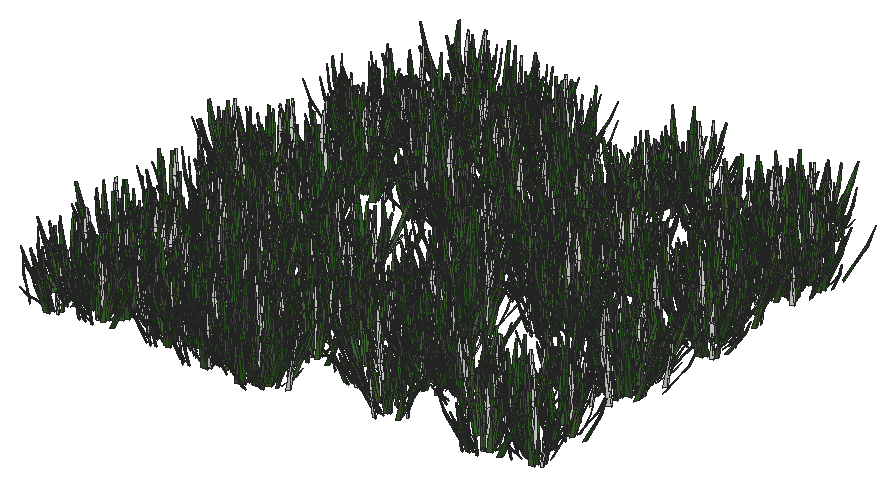
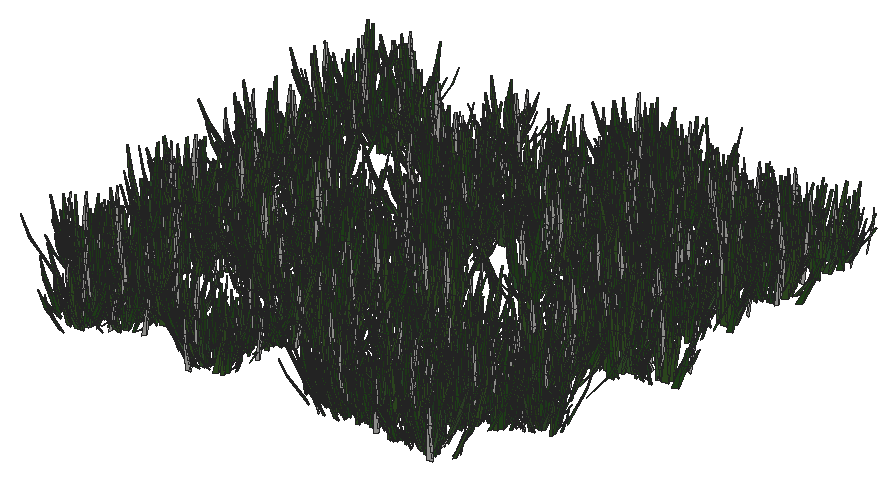
# SketchUp Ruby script. Lengths in inches.
U = 1.inch
M = Sketchup.active_model
def pt(a) = Geom::Point3d.new(a.map { |v| v * U })
def face(e, loops, mat)
  f = e.add_face(loops[0].map { |a| pt(a) })
  loops[1..].each { |l| e.add_face(l.map { |a| pt(a) }).erase! }
  f.material = f.back_material = mat if mat
  f
end
# faces: each face lists its corners as indices into pts; further lists are holes
def faces(e, pts, list, mat = nil) = list.each { |f| face(e, (f[0].is_a?(Array) ? f : [f]).map { |l| l.map { |i| pts[i] } }, mat) }
# xy, xz, yz: faces in a plane at the given z, y or x. An outline is a flat list of corners, or four numbers for a rectangle; further outlines are holes
def ring(l) = l.size == 4 ? [[l[0], l[1]], [l[2], l[1]], [l[2], l[3]], [l[0], l[3]]] : l.each_slice(2).to_a
def flat(e, list, mat, &to3) = list.each { |f| face(e, (f[0].is_a?(Array) ? f : [f]).map { |l| ring(l).map { |u, v| to3.(u, v) } }, mat) }
def xy(e, z, list, mat = nil) = flat(e, list, mat) { |x, y| [x, y, z] }
def xz(e, y, list, mat = nil) = flat(e, list, mat) { |x, z| [x, y, z] }
def yz(e, x, list, mat = nil) = flat(e, list, mat) { |y, z| [x, y, z] }
def lines(e, pts, list) = list.each { |a, b| e.add_line(pt(pts[a]), pt(pts[b])) }
# prism: a flat outline (further loops are holes) pulled along v
def prism(e, loops, v, mat = nil)
  f = face(e, loops, mat); d = Geom::Vector3d.new(v.map { |x| x * U })
  f.pushpull(f.normal.samedirection?(d) ? d.length : -d.length)
end
def box(e, o, s, mat = nil) = prism(e, [[o, [o[0] + s[0], o[1], o[2]], [o[0] + s[0], o[1] + s[1], o[2]], [o[0], o[1] + s[1], o[2]]]], [0, 0, s[2]], mat)
def at(x, y, z, deg = 0) = Geom::Transformation.translation(pt([x, y, z])) * Geom::Transformation.rotation(ORIGIN, Z_AXIS, deg.degrees)
def axes(o, x, y, z) = Geom::Transformation.new([*x, 0, *y, 0, *z, 0, *pt(o).to_a, 1])
def part(name) = M.definitions.add(name)
# library, detail: a bought-in or finely detailed component or shape, given as its bounding box
def library(name, o, s) = part(name).tap { |d| box(d.entities, o, s) }
def detail(e, o, s) = box(e.add_group.entities, o, s)
def put(e, d, t, mat = nil) = e.add_instance(d, t).tap { |i| i.material = mat if mat }
def group(e, t, mat = nil) = e.add_group.tap { |g| g.transformation = t; g.material = mat if mat }.entities
root = M.entities
M.materials.add("Material1").color = [58, 110, 58]
M.materials.add("Material10").color = [48, 100, 38]
M.materials.add("Material3").color = [68, 110, 58]
M.materials.add("Material4").color = [48, 90, 38]
M.materials.add("Material5").color = [68, 110, 48]
M.materials.add("Material6").color = [48, 90, 48]
M.materials.add("Material8").color = [58, 90, 38]
M.materials.add("Material9").color = [68, 100, 58]
c1 = part("grass00")
p = [[-0.6875,0.15,0],[-0.56,0.08,5.52],[-0.04,0.03,2.76],[0.48,-0.02,0],[0.35,-0.02,5.52],[-0.1,-0.14,5.52],
  [-0.12,0.65,8.37],[-0.42,0.65,8.37]]
faces(c1.entities,p,[[0,1,2,3],[3,2,4],[1,5,2],[5,4,2],[1,6,5],[4,5,6],[7,6,1]])
c2 = part("Group16\#1")
put(c2.entities,c1,axes([1.44,-0.61,-0.01],[0.05352,0.12609,0],[-0.10704,0.04543,0.07239],[0.06664,-0.02828,0.11628]),"Material6")
put(c2.entities,c1,axes([0.76,-0.15,-0.01],[0.04676,0.24062,0],[-0.23162,0.04501,0.06642],[0.0652,-0.01267,0.23595]),"Material3")
put(c2.entities,c1,axes([0.79,0.01,-0.01],[-0.00606,0.34651,0],[-0.34381,-0.00602,0.0432],[0.04319,0.00076,0.34386]))
put(c2.entities,c1,axes([1,0.23,-0.01],[-0.07192,0.31144,0],[-0.28722,-0.06632,0.1236],[0.12043,0.02781,0.29478]),"Material5")
put(c2.entities,c1,axes([1.66,0.77,-0.01],[-0.13828,0.29651,0],[-0.21551,-0.1005,0.22471],[0.20365,0.09498,0.23779]),"Material10")
put(c2.entities,c1,axes([0.6875,0.52,-0.01],[-0.18126,0.24051,0],[-0.22746,-0.17142,0.09788],[0.07817,0.05891,0.28481]),"Material5")
put(c2.entities,c1,axes([0.68,0.78,-0.01],[-0.215,0.18688,0],[-0.12385,-0.14248,0.21334],[0.13995,0.16101,0.18878]),"Material3")
put(c2.entities,c1,axes([0.56,1,-0.01],[-0.13756,0.07624,0],[-0.06159,-0.11112,0.0927],[0.04494,0.08108,0.12705]),"Material5")
put(c2.entities,c1,axes([0.2,0.64,-0.01],[-0.23729,0.07254,0],[-0.05711,-0.18681,0.153],[0.04473,0.14632,0.19535]),"Material10")
put(c2.entities,c1,axes([0.0625,0.72,-0.01],[-0.28874,0.02525,0],[-0.02179,-0.24916,0.14647],[0.01276,0.14591,0.25012]),"Material3")
put(c2.entities,c1,axes([-0.08,0.62,-0.01],[-0.34089,-0.04187,0],[0.03255,-0.26504,0.216],[-0.02633,0.21439,0.26703]),"Material10")
put(c2.entities,c1,axes([-0.34,0.98,-0.01],[-0.14314,-0.0493,0],[0.04397,-0.12769,0.06843],[-0.02228,0.0647,0.13505]),"Material10")
put(c2.entities,c1,axes([-0.87,1.45,-0.01],[-0.23488,-0.14114,0],[0.13761,-0.22901,0.06087],[-0.03135,0.05217,0.26717]))
put(c2.entities,c1,axes([-0.72,0.77,-0.01],[-0.14208,-0.13251,0],[0.07209,-0.0773,0.16301],[-0.11118,0.11922,0.1057]),"Material10")
put(c2.entities,c1,axes([-0.62,0.43,-0.01],[-0.14845,-0.21203,0],[0.18654,-0.13061,0.12304],[-0.10079,0.07057,0.22772]),"Material3")
put(c2.entities,c1,axes([-0.68,0.29,-0.01],[-0.13639,-0.32136,0],[0.31723,-0.13464,0.05579],[-0.05136,0.0218,0.34462]),"Material4")
put(c2.entities,c1,axes([-0.64,0.125,-0.01],[-0.0458,-0.23569,0],[0.22124,-0.043,0.08276],[-0.08124,0.01579,0.22538]),"Material1")
put(c2.entities,c1,axes([-1.6,-0.03,-0.01],[0.00576,-0.32897,0],[0.27526,0.00482,0.18018],[-0.18015,-0.00315,0.2753]),"Material5")
put(c2.entities,c1,axes([-1.36,-0.31,-0.01],[0.05718,-0.24765,0],[0.18172,0.04196,0.17267],[-0.16825,-0.03885,0.1865]),"Material10")
put(c2.entities,c1,axes([-1.54,-0.72,-0.01],[0.06537,-0.14017,0],[0.13555,0.06321,0.03939],[-0.0357,-0.01665,0.14956]))
put(c2.entities,c1,axes([-1.19,-0.9,-0.01],[0.09597,-0.12735,0],[0.11214,0.08451,0.07557],[-0.06035,-0.04548,0.14042]),"Material9")
put(c2.entities,c1,axes([-0.47,-0.54,-0.01],[0.11588,-0.10072,0],[0.0618,0.0711,0.12124],[-0.07953,-0.0915,0.0942]))
put(c2.entities,c1,axes([-0.47,-0.84,-0.01],[0.11927,-0.0661,0],[0.06603,0.11913,0.00646],[-0.00313,-0.00565,0.13621]),"Material5")
put(c2.entities,c1,axes([-0.38,-1.24,-0.01],[0.28037,-0.08571,0],[0.0618,0.20215,0.20315],[-0.05939,-0.19428,0.21139]),"Material9")
put(c2.entities,c1,axes([-0.06,-0.66,-0.01],[0.22719,-0.01987,0],[0.01247,0.14255,0.17758],[-0.01547,-0.17691,0.1431]),"Material8")
put(c2.entities,c1,axes([0.11,-0.89,-0.01],[0.14882,0.01828,0],[-0.01058,0.08611,0.12229],[0.01491,-0.12138,0.08676]),"Material6")
put(c2.entities,c1,axes([0.25,-0.72,-0.01],[0.20481,0.07053,0],[-0.06206,0.18022,0.10291],[0.03351,-0.0973,0.1906]),"Material6")
put(c2.entities,c1,axes([0.85,-1.42,-0.01],[0.16481,0.09904,0],[-0.09472,0.15762,0.05616],[0.02893,-0.04814,0.18389]),"Material5")
put(c2.entities,c1,axes([1.01,-1.09,-0.01],[0.21858,0.20385,0],[-0.17495,0.1876,0.15339],[0.10462,-0.11218,0.25652]),"Material10")
put(c2.entities,c1,axes([1.01,-0.71,-0.01],[0.08733,0.12473,0],[-0.06445,0.04512,0.13037],[0.1068,-0.07477,0.07867]),"Material6")
c3 = part("Group15\#1")
put(c3.entities,c2,at(0,0,0))
c4 = part("3darcstudiotree_grass00\#1")
put(c4.entities,c3,at(0,0,0))
put(root,c4,axes([313.43,128.25,0.25],[1.09323,-0.33647,0],[0.38565,0.86321,-0.01564],[0.00925,0.0207,1.88746]))
put(root,c4,axes([302.23,128.25,0.25],[0.61135,-0.6937,0],[0.76743,0.46592,-0.02877],[0.03641,0.02211,1.49076]))
put(root,c4,axes([310.46,128.14,0.25],[0.83193,0.6505,0],[-0.85398,0.75239,-0.01047],[-0.01109,0.00977,1.92288]))
put(root,c4,axes([314.96,128.14,0.25],[-0.65984,-0.73253,0],[0.79893,-0.49577,-0.02089],[0.02661,-0.01651,1.58683]))
put(root,c4,axes([299.16,128.03,0.25],[-0.33379,1.0049,0],[-0.95038,-0.21747,-0.03305],[-0.04366,-0.00999,1.35106]))
put(root,c4,axes([307.23,128.39,0.25],[0.52907,0.62243,0],[-0.7421,0.43455,-0.03223],[-0.03993,0.02338,1.37708]))
put(root,c4,axes([301.17,128.74,0.25],[1.04664,0.25601,0],[-0.25703,0.72391,-0.026],[-0.0129,0.03632,1.59572]))
put(root,c4,axes([311.2,128.65,0.25],[-1.02803,0.5315,0],[-0.48139,-0.64144,-0.01072],[-0.0115,-0.01532,1.84718]))
put(root,c4,axes([302.79,129.78,0.25],[1.1255,0.00235,0],[-0.00289,0.95262,-0.01268],[-0.00005,0.01678,1.83013]))
put(root,c4,axes([329.86,130.03,0.25],[0.62937,-0.55545,0],[0.77494,0.60491,-0.02136],[0.02372,0.01851,1.62144]))
put(root,c4,axes([310.44,129.93,0.25],[0.78925,0.37102,0],[-0.48273,0.70741,-0.02459],[-0.02361,0.0346,1.90817]))
put(root,c4,axes([299.36,129.74,0.25],[-0.10935,0.97509,0],[-1.19512,-0.09233,-0.02425],[-0.03553,-0.00274,1.76617]))
put(root,c4,axes([301.375,129.97,0.25],[0.27214,0.80157,0],[-1.04551,0.24453,-0.02067],[-0.03104,0.00726,1.69495]))
put(root,c4,axes([307.62,129.96,0.25],[0.12593,0.77017,0],[-0.97904,0.11028,-0.02967],[-0.04682,0.00527,1.57371]))
put(root,c4,axes([322.625,130.01,0.25],[-0.84483,0.43279,0],[-0.48176,-0.64786,-0.03387],[-0.02627,-0.03533,1.3548]))
put(root,c4,axes([305.28,130.84,0.25],[-0.84379,0.61822,0],[-0.85319,-0.80223,-0.01862],[-0.01823,-0.01715,1.90809]))
put(root,c4,axes([332.8125,131.04,0.25],[-0.49439,0.70839,0],[-0.82415,-0.39624,-0.02138],[-0.03174,-0.01526,1.63406]))
put(root,c4,axes([313.39,131.35,0.25],[-0.70228,-0.48257,0],[0.74708,-0.74899,-0.02106],[0.01665,-0.01669,1.45262]))
put(root,c4,axes([306.87,131.27,0.25],[-0.85735,0.46398,0],[-0.6008,-0.76479,-0.02083],[-0.01661,-0.02115,1.60618]))
put(root,c4,axes([301.49,131.9,0.25],[-0.71478,-0.65935,0],[0.79567,-0.59421,-0.02928],[0.02765,-0.02065,1.35967]))
put(root,c4,axes([311.6,132.11,0.25],[0.18112,-1.06483,0],[1.06399,0.12468,-0.01886],[0.0303,0.00355,1.74385]))
put(root,c4,axes([310.375,132.125,0.25],[1.08899,0.1057,0],[-0.112,0.79493,-0.0104],[-0.00234,0.01663,1.87036]))
put(root,c4,axes([304.09,132.35,0.25],[1.13568,-0.03992,0],[0.04696,0.92039,-0.02002],[0.00129,0.02535,1.69539]))
put(root,c4,axes([314.64,132.64,0.25],[0.8623,-0.69628,0],[0.62912,0.53673,-0.01443],[0.02081,0.01775,1.86565]))
put(root,c4,axes([318.99,132.49,0.25],[0.11272,1.05535,0],[-1.08573,0.07989,-0.0152],[-0.02232,0.00164,1.60635]))
put(root,c4,axes([322.37,133.39,0.25],[0.89828,0.57164,0],[-0.56596,0.61268,-0.03117],[-0.02658,0.02877,1.30357]))
put(root,c4,axes([325.61,133.9,0.25],[0.03302,-0.91614,0],[1.14545,0.02844,-0.01737],[0.02345,0.00058,1.54781]))
put(root,c4,axes([301.54,133.72,0.25],[-0.15265,0.9589,0],[-1.24925,-0.137,-0.03274],[-0.03717,-0.00408,1.44297]))
put(root,c4,axes([329.42,134.3,0.25],[0.89818,-0.35172,0],[0.49737,0.87499,-0.02435],[0.01511,0.02658,1.69455]))
put(root,c4,axes([311.57,133.92,0.25],[-1.14214,-0.02536,0],[0.03102,-0.96222,-0.01377],[0.00052,-0.01628,1.65227]))
put(root,c4,axes([299.1875,133.91,0.25],[-0.79807,0.55513,0],[-0.82006,-0.81217,-0.01682],[-0.01524,-0.01509,1.80026]))
put(root,c4,axes([332.37,134.4375,0.25],[0.86483,-0.466,0],[0.52618,0.67271,-0.02789],[0.02695,0.03446,1.71527]))
put(root,c4,axes([328.21,134.33,0.25],[-0.98544,0.42877,0],[-0.41843,-0.66251,-0.02232],[-0.01829,-0.02895,1.59039]))
put(root,c4,axes([302.13,134.41,0.25],[0.21228,0.86046,0],[-1.13808,0.19343,-0.02758],[-0.03776,0.00642,1.62317]))
put(root,c4,axes([299.88,134.7,0.25],[0.63523,0.53865,0],[-0.7856,0.63824,-0.01876],[-0.02159,0.01754,1.77063]))
put(root,c4,axes([309.61,135.07,0.25],[-0.08387,-0.77908,0],[1.1557,-0.08571,-0.01785],[0.02919,-0.00216,1.90542]))
put(root,c4,axes([320.69,134.98,0.25],[0.93635,0.57595,0],[-0.61403,0.6877,-0.03152],[-0.02685,0.03007,1.47514]))
put(root,c4,axes([321.74,135.15,0.25],[0.073,0.99528,0],[-1.03512,0.05231,-0.02381],[-0.04076,0.00206,1.77807]))
put(root,c4,axes([306.58,135.61,0.25],[-0.50394,-0.92094,0],[1.07294,-0.40446,-0.02239],[0.03283,-0.01238,1.89813]))
put(root,c4,axes([311.75,135.85,0.25],[1.04801,-0.5177,0],[0.58045,0.80949,-0.02674],[0.01812,0.02528,1.50406]))
put(root,c4,axes([305.66,136.03,0.25],[1.1531,0.08555,0],[-0.0892,0.82822,-0.01038],[-0.00179,0.01662,1.94021]))
put(root,c4,axes([308.67,135.98,0.25],[-0.82708,-0.3732,0],[0.44077,-0.67293,-0.02167],[0.01498,-0.02287,1.33527]))
put(root,c4,axes([322.77,135.96,0.25],[-1.19556,-0.39954,0],[0.44888,-0.92534,-0.01703],[0.00869,-0.01792,1.64249]))
put(root,c4,axes([314.28,136.01,0.25],[-1.04881,0.00914,0],[-0.01096,-0.86641,-0.01485],[-0.00024,-0.01921,1.62647]))
put(root,c4,axes([315.67,136.35,0.25],[-0.59415,-0.84264,0],[0.77882,-0.37831,-0.0221],[0.03853,-0.01871,1.82262]))
put(root,c4,axes([320.71,136.86,0.25],[-0.68329,-0.49168,0],[0.59227,-0.56702,-0.00893],[0.01284,-0.0123,1.98619]))
put(root,c4,axes([304.01,137.55,0.25],[0.3214,-0.86698,0],[1.22076,0.31177,-0.02541],[0.02819,0.0072,1.48254]))
put(root,c4,axes([312.76,137.57,0.25],[1.11449,-0.25107,0],[0.30887,0.94451,-0.0215],[0.00816,0.02495,1.70776]))
put(root,c4,axes([330.19,138.15,0.25],[-0.63388,-0.55014,0],[0.76625,-0.60822,-0.03327],[0.0297,-0.02357,1.30962]))
put(root,c4,axes([302.79,138.39,0.25],[0.24456,-1.04334,0],[1.1039,0.17825,-0.02432],[0.03295,0.00532,1.55217]))
put(root,c4,axes([313.18,138.2,0.25],[-0.83238,0.61366,0],[-0.6415,-0.59945,-0.02123],[-0.02,-0.01868,1.37003]))
put(root,c4,axes([299.72,138.37,0.25],[-0.44738,0.79737,0],[-0.90216,-0.3487,-0.01596],[-0.02712,-0.01048,1.86544]))
put(root,c4,axes([305.69,138.7,0.25],[0.30388,0.87562,0],[-0.98281,0.23497,-0.02733],[-0.04221,0.01009,1.64375]))
put(root,c4,axes([316.1,138.91,0.25],[-0.59845,-0.67902,0],[0.85359,-0.51827,-0.02018],[0.02788,-0.01693,1.81061]))
put(root,c4,axes([318.25,139.49,0.25],[-1.06497,-0.45043,0],[0.57917,-0.94334,-0.02171],[0.01216,-0.01981,1.57387]))
put(root,c4,axes([302.68,139.47,0.25],[-1.28573,0.12644,0],[-0.12594,-0.88224,-0.03012],[-0.00432,-0.03026,1.30483]))
put(root,c4,axes([319.02,139.47,0.25],[-0.97202,0.52359,0],[-0.55407,-0.70861,-0.02727],[-0.02059,-0.02633,1.41127]))
put(root,c4,axes([328.27,139.66,0.25],[-0.78533,-0.41804,0],[0.53335,-0.69026,-0.01822],[0.0159,-0.02058,1.59761]))
put(root,c4,axes([311.28,139.7,0.25],[-0.77915,0.67604,0],[-0.83871,-0.66591,-0.01205],[-0.01406,-0.01117,1.87482]))
put(root,c4,axes([331.87,140.01,0.25],[-1.05758,0.07034,0],[-0.1014,-1.05028,-0.02116],[-0.00239,-0.02472,1.79229]))
put(root,c4,axes([320.61,140.79,0.25],[1.15762,-0.3893,0],[0.44335,0.90821,-0.01357],[0.00856,0.01754,1.98263]))
put(root,c4,axes([307.64,140.73,0.25],[-0.82934,0.77217,0],[-0.7456,-0.55167,-0.02096],[-0.02632,-0.01947,1.6805]))
put(root,c4,axes([331.89,141.28,0.25],[1.26498,-0.20882,0],[0.25155,1.04976,-0.02703],[0.007,0.02922,1.71263]))
put(root,c4,axes([300.78,140.9,0.25],[-1.05239,-0.22175,0],[0.29558,-0.96637,-0.00944],[0.00374,-0.01223,1.93444]))
put(root,c4,axes([305.27,141.21,0.25],[-0.59651,0.64086,0],[-0.89795,-0.57578,-0.01374],[-0.01625,-0.01042,1.69563]))
put(root,c4,axes([331.8,142.09,0.25],[-0.58332,-0.95918,0],[1.04759,-0.43889,-0.02075],[0.02643,-0.01107,1.67433]))
put(root,c4,axes([316.4,142.55,0.25],[1.13433,-0.26746,0],[0.2742,0.80112,-0.02465],[0.00948,0.0277,1.41248]))
put(root,c4,axes([302.11,142.33,0.25],[-0.88118,0.22893,0],[-0.36633,-0.97138,-0.0251],[-0.00976,-0.02587,1.59541]))
put(root,c4,axes([317.5625,143.43,0.25],[0.97422,0.44789,0],[-0.5681,0.85127,-0.02111],[-0.01665,0.02494,1.90804]))
put(root,c4,axes([324.09,143.39,0.25],[0.5727,0.59367,0],[-0.78662,0.52276,-0.01526],[-0.02308,0.01534,1.9517]))
put(root,c4,axes([310.62,143.41,0.25],[-1.28434,-0.13842,0],[0.15763,-1.00753,-0.02421],[0.00423,-0.02702,1.66024]))
put(root,c4,axes([301.36,143.76,0.25],[-0.03552,-0.88054,0],[1.15993,-0.03223,-0.02714],[0.03379,-0.00094,1.44559]))
put(root,c4,axes([331.49,143.48,0.25],[-0.83739,0.6212,0],[-0.76277,-0.70835,-0.02716],[-0.02098,-0.01948,1.32671]))
put(root,c4,axes([303.99,143.74,0.25],[-0.79211,-0.5677,0],[0.64124,-0.61637,-0.01919],[0.02549,-0.0245,1.99409]))
put(root,c4,axes([317.37,144.68,0.25],[1.00024,-0.28864,0],[0.34212,0.81672,-0.02118],[0.01157,0.02761,1.73224]))
put(root,c4,axes([326.71,144.67,0.25],[-1.02537,-0.31244,0],[0.35342,-0.79903,-0.02574],[0.01198,-0.02708,1.38465]))
put(root,c4,axes([305.08,144.86,0.25],[0.88915,0.70681,0],[-0.86796,0.75219,-0.01961],[-0.01791,0.01552,1.65716]))
put(root,c4,axes([325.1,144.92,0.25],[-0.23063,-0.72462,0],[1.18922,-0.26075,-0.01354],[0.02028,-0.00445,1.90468]))
put(root,c4,axes([320.89,146,0.25],[0.6968,0.64746,0],[-0.69574,0.51582,-0.01423],[-0.0208,0.01542,1.82816]))
put(root,c4,axes([316.8,146.18,0.25],[0.94145,0.15722,0],[-0.18431,0.7603,-0.0192],[-0.00666,0.02747,1.64321]))
put(root,c4,axes([298.19,146.02,0.25],[-0.51854,0.6931,0],[-0.98757,-0.50899,-0.02009],[-0.02474,-0.01275,1.68525]))
put(root,c4,axes([314.57,146.4,0.25],[0.75471,0.45208,0],[-0.71294,0.81993,-0.01696],[-0.01498,0.01722,1.8379]))
put(root,c4,axes([300.56,146.24,0.25],[0.295,0.86172,0],[-1.1428,0.26951,-0.01918],[-0.02926,0.0069,1.88463]))
put(root,c4,axes([329.91,146.22,0.25],[-0.47274,0.64498,0],[-1.00249,-0.50619,-0.02284],[-0.02735,-0.01381,1.64481]))
put(root,c4,axes([315.74,147,0.25],[1.12211,-0.08267,0],[0.10176,0.95149,-0.01913],[0.00274,0.02558,1.86132]))
put(root,c4,axes([301.28,146.88,0.25],[-0.03917,0.82453,0],[-1.18535,-0.03879,-0.01193],[-0.01988,-0.00065,1.97773]))
put(root,c4,axes([323.37,147.27,0.25],[0.4609,-0.8182,0],[1.06881,0.41476,-0.01397],[0.01867,0.00725,1.74087]))
put(root,c4,axes([304.1,147.23,0.25],[-0.76517,0.77215,0],[-0.95428,-0.65146,-0.01702],[-0.02035,-0.01389,1.91367]))
put(root,c4,axes([332.68,147.55,0.25],[-0.26517,0.76227,0],[-1.14223,-0.27373,-0.01983],[-0.02316,-0.00555,1.44555]))
put(root,c4,axes([303.0625,148.12,0.25],[0.96269,-0.20808,0],[0.25812,0.82269,-0.03218],[0.01045,0.03332,1.32043]))
put(root,c4,axes([316.76,148.49,0.25],[-1.24601,0.07432,0],[-0.0817,-0.94358,-0.01837],[-0.00177,-0.02047,1.53349]))
put(root,c4,axes([331.13,148.96,0.25],[0.63478,-0.71481,0],[1.02472,0.62689,-0.00987],[0.01189,0.00727,1.9048]))
put(root,c4,axes([314.26,148.56,0.25],[-0.70982,0.78602,0],[-0.93962,-0.58455,-0.01976],[-0.0234,-0.01455,1.7373]))
put(root,c4,axes([331.73,149.42,0.25],[0.35992,0.76837,0],[-1.16931,0.37733,-0.01993],[-0.02949,0.00952,1.99239]))
put(root,c4,axes([319.41,149.65,0.25],[-1.09359,-0.43693,0],[0.40459,-0.69761,-0.01121],[0.00989,-0.01705,1.89718]))
put(root,c4,axes([311.65,149.55,0.25],[-0.48144,0.69691,0],[-1.01289,-0.48204,-0.01882],[-0.02723,-0.01296,1.94745]))
put(root,c4,axes([309.06,149.88,0.25],[-0.1303,0.90117,0],[-0.89358,-0.089,-0.01529],[-0.02819,-0.00281,1.67142]))
put(root,c4,axes([305.11,149.97,0.25],[-0.82871,0.72762,0],[-0.79242,-0.62174,-0.01805],[-0.0206,-0.01617,1.71251]))
put(root,c4,axes([316.47,150.21,0.25],[-0.53132,0.65289,0],[-1.06151,-0.59511,-0.01862],[-0.0227,-0.01273,1.88514]))
put(root,c4,axes([324.1,150.65,0.25],[0.32675,-0.77404,0],[1.18652,0.34506,-0.02001],[0.02666,0.00775,1.77455]))
put(root,c4,axes([325.13,150.21,0.25],[-0.68507,0.59882,0],[-0.92124,-0.72604,-0.01749],[-0.01788,-0.01409,1.7911]))
put(root,c4,axes([304.09,150.84,0.25],[1.17385,0.4283,0],[-0.44026,0.83126,-0.02572],[-0.01392,0.02628,1.47108]))
put(root,c4,axes([325.0625,150.88,0.25],[-0.77624,0.54618,0],[-0.68304,-0.66875,-0.0209],[-0.01895,-0.01855,1.48072]))
put(root,c4,axes([302.0625,151.1,0.25],[-1.1556,0.1687,0],[-0.16771,-0.7914,-0.03096],[-0.00769,-0.03628,1.38775]))
put(root,c4,axes([311.87,151.43,0.25],[0.69908,0.60878,0],[-0.92641,0.73286,-0.0237],[-0.01811,0.01432,1.35093]))
put(root,c4,axes([319.72,151.49,0.25],[1.1842,0.39183,0],[-0.34588,0.72011,-0.02018],[-0.01107,0.02305,1.38364]))
put(root,c4,axes([331.75,151.39,0.25],[-1.07973,0.19755,0],[-0.21759,-0.81928,-0.01188],[-0.00505,-0.01902,1.99665]))
put(root,c4,axes([326.875,151.91,0.25],[0.13038,-1.03831,0],[0.92657,0.08015,-0.02929],[0.04877,0.00422,1.55926]))
put(root,c4,axes([303.125,152.3,0.25],[0.97403,-0.13367,0],[0.20627,1.03542,-0.01648],[0.00323,0.01622,1.51991]))
put(root,c4,axes([323.53,152.61,0.25],[-0.66717,-0.52576,0],[0.75675,-0.66154,-0.01822],[0.02133,-0.01865,1.86907]))
put(root,c4,axes([317.48,152.69,0.25],[-1.17262,0.24748,0],[-0.23585,-0.76983,-0.01716],[-0.00828,-0.02704,1.87475]))
put(root,c4,axes([321.32,153.36,0.25],[0.42227,-0.80225,0],[1.10309,0.4,-0.02716],[0.03033,0.011,1.46706]))
put(root,c4,axes([328.29,153.4,0.25],[0.86588,-0.51585,0],[0.52509,0.60719,-0.02763],[0.02372,0.02743,1.3256]))
put(root,c4,axes([316.37,153.41,0.25],[-1.05948,0.58075,0],[-0.60306,-0.75792,-0.01955],[-0.01446,-0.01818,1.46911]))
put(root,c4,axes([330.02,153.76,0.25],[-0.52155,-0.71373,0],[0.89543,-0.45077,-0.01057],[0.01599,-0.00805,1.85267]))
put(root,c4,axes([311.53,154.5,0.25],[1.1938,0.12032,0],[-0.11678,0.7982,-0.01966],[-0.00437,0.02988,1.78732]))
put(root,c4,axes([328.6875,154.88,0.25],[-0.24128,-0.97226,0],[1.00526,-0.17186,-0.02826],[0.04297,-0.00735,1.59374]))
put(root,c4,axes([306.7,154.59,0.25],[-0.80264,0.48827,0],[-0.72231,-0.81798,-0.02359],[-0.01906,-0.02158,1.66971]))
put(root,c4,axes([300.67,155.01,0.25],[-0.25337,-0.83383,0],[1.02151,-0.21384,-0.02503],[0.03406,-0.00713,1.47852]))
put(root,c4,axes([317.89,155.03,0.25],[-0.31549,-0.96475,0],[0.99962,-0.2252,-0.0298],[0.03984,-0.00897,1.43464]))
put(root,c4,axes([331.43,154.89,0.25],[0.23523,0.919,0],[-1.00659,0.17749,-0.01067],[-0.01856,0.00327,1.82972]))
put(root,c4,axes([305.95,155.07,0.25],[0.50931,0.77706,0],[-0.81187,0.36658,-0.01685],[-0.031,0.014,1.93576]))
put(root,c4,axes([300.08,155.19,0.25],[-0.87857,-0.37897,0],[0.41615,-0.66464,-0.02241],[0.0193,-0.03083,1.68548]))
put(root,c4,axes([310.05,155.97,0.25],[1.03934,-0.18857,0],[0.22666,0.86064,-0.02018],[0.0061,0.02318,1.50307]))
put(root,c4,axes([332.52,155.71,0.25],[-0.89254,-0.12533,0],[0.15833,-0.7768,-0.02254],[0.00552,-0.02709,1.39425]))
put(root,c4,axes([314.8,155.86,0.25],[-0.55854,-0.60247,0],[0.86141,-0.55016,-0.03027],[0.0326,-0.02082,1.47708]))
put(root,c4,axes([304.01,156.36,0.25],[0.00119,-0.83737,0],[1.03275,0.00101,-0.01884],[0.02654,0.00003,1.45492]))
put(root,c4,axes([317.95,156.12,0.25],[-0.7731,0.48149,0],[-0.73459,-0.81255,-0.02868],[-0.01955,-0.02162,1.39]))
put(root,c4,axes([302.67,156.28,0.25],[-1.12467,-0.02722,0],[0.02702,-0.76927,-0.0193],[0.00121,-0.03446,1.99558]))
put(root,c4,axes([307.05,157.39,0.25],[0.88333,-0.29816,0],[0.36293,0.74073,-0.02601],[0.01495,0.03052,1.4702]))
put(root,c4,axes([319.19,157.24,0.25],[0.49895,0.95979,0],[-1.13466,0.40635,-0.02206],[-0.02696,0.00966,1.64521]))
put(root,c4,axes([332.36,157.67,0.25],[1.15497,0.32051,0],[-0.31783,0.789,-0.01696],[-0.00972,0.02413,1.81122]))
put(root,c4,axes([304,157.42,0.25],[-1.00274,0.40134,0],[-0.43065,-0.74124,-0.02015],[-0.01665,-0.02867,1.88684]))
put(root,c4,axes([305.19,157.78,0.25],[0.17738,1.02916,0],[-1.18429,0.14062,-0.02596],[-0.02849,0.00338,1.32635]))
put(root,c4,axes([331.48,158.32,0.25],[0.96421,-0.60452,0],[0.56864,0.62483,-0.01203],[0.01474,0.01619,1.91781]))
put(root,c4,axes([325.39,158.52,0.25],[0.27804,-0.80219,0],[1.14819,0.27416,-0.0144],[0.02093,0.005,1.80693]))
put(root,c4,axes([328.03,158.72,0.25],[1.14497,-0.13365,0],[0.174,1.02686,-0.01318],[0.00292,0.01722,1.98636]))
put(root,c4,axes([323.94,158.82,0.25],[0.95384,0.11491,0],[-0.17429,0.99664,-0.0224],[-0.00376,0.02149,1.41716]))
put(root,c4,axes([319.76,158.86,0.25],[0.75747,0.54232,0],[-0.73181,0.70415,-0.02494],[-0.02378,0.02288,1.63549]))
put(root,c4,axes([327.125,159.04,0.25],[0.363,-0.93176,0],[0.95549,0.25644,-0.02554],[0.03399,0.00912,1.40467]))
put(root,c4,axes([312.78,159.43,0.25],[-0.84106,0.76206,0],[-0.81648,-0.62079,-0.02313],[-0.0298,-0.02266,1.93523]))
put(root,c4,axes([310.63,159.61,0.25],[0.32106,0.98302,0],[-1.02938,0.23161,-0.02312],[-0.03146,0.00708,1.50331]))
put(root,c4,axes([311.37,160.28,0.25],[0.95241,0.40171,0],[-0.56791,0.92756,-0.02666],[-0.0143,0.02335,1.48409]))
put(root,c4,axes([308.1875,160.89,0.25],[0.94276,0.15446,0],[-0.19421,0.81661,-0.02055],[-0.00745,0.03131,1.87683]))
put(root,c4,axes([305.85,160.7,0.25],[-0.96994,0.58419,0],[-0.60673,-0.69397,-0.01293],[-0.01414,-0.01618,1.92389]))
put(root,c4,axes([326.82,161.06,0.25],[0.70849,0.64738,0],[-0.75672,0.57051,-0.01914],[-0.01968,0.01483,1.41957]))
put(root,c4,axes([319.54,160.95,0.25],[-0.8953,-0.15066,0],[0.24291,-0.9944,-0.02938],[0.00631,-0.02583,1.3208]))
put(root,c4,axes([310.07,161.11,0.25],[-0.96147,-0.41544,0],[0.49541,-0.78986,-0.02288],[0.01509,-0.02405,1.53217]))
put(root,c4,axes([328.75,161.4,0.25],[0.90457,-0.25622,0],[0.30614,0.74459,-0.02189],[0.01388,0.03375,1.86062]))
put(root,c4,axes([303.54,161.4,0.25],[1.27559,-0.03418,0],[0.0322,0.82791,-0.01793],[0.00104,0.02673,1.79317]))
put(root,c4,axes([320.39,161.57,0.25],[0.9155,-0.45305,0],[0.55155,0.76781,-0.01626],[0.01396,0.01943,1.80561]))
put(root,c4,axes([328.93,162.23,0.25],[0.6194,0.89163,0],[-0.94156,0.4506,-0.02249],[-0.02914,0.01395,1.62577]))
